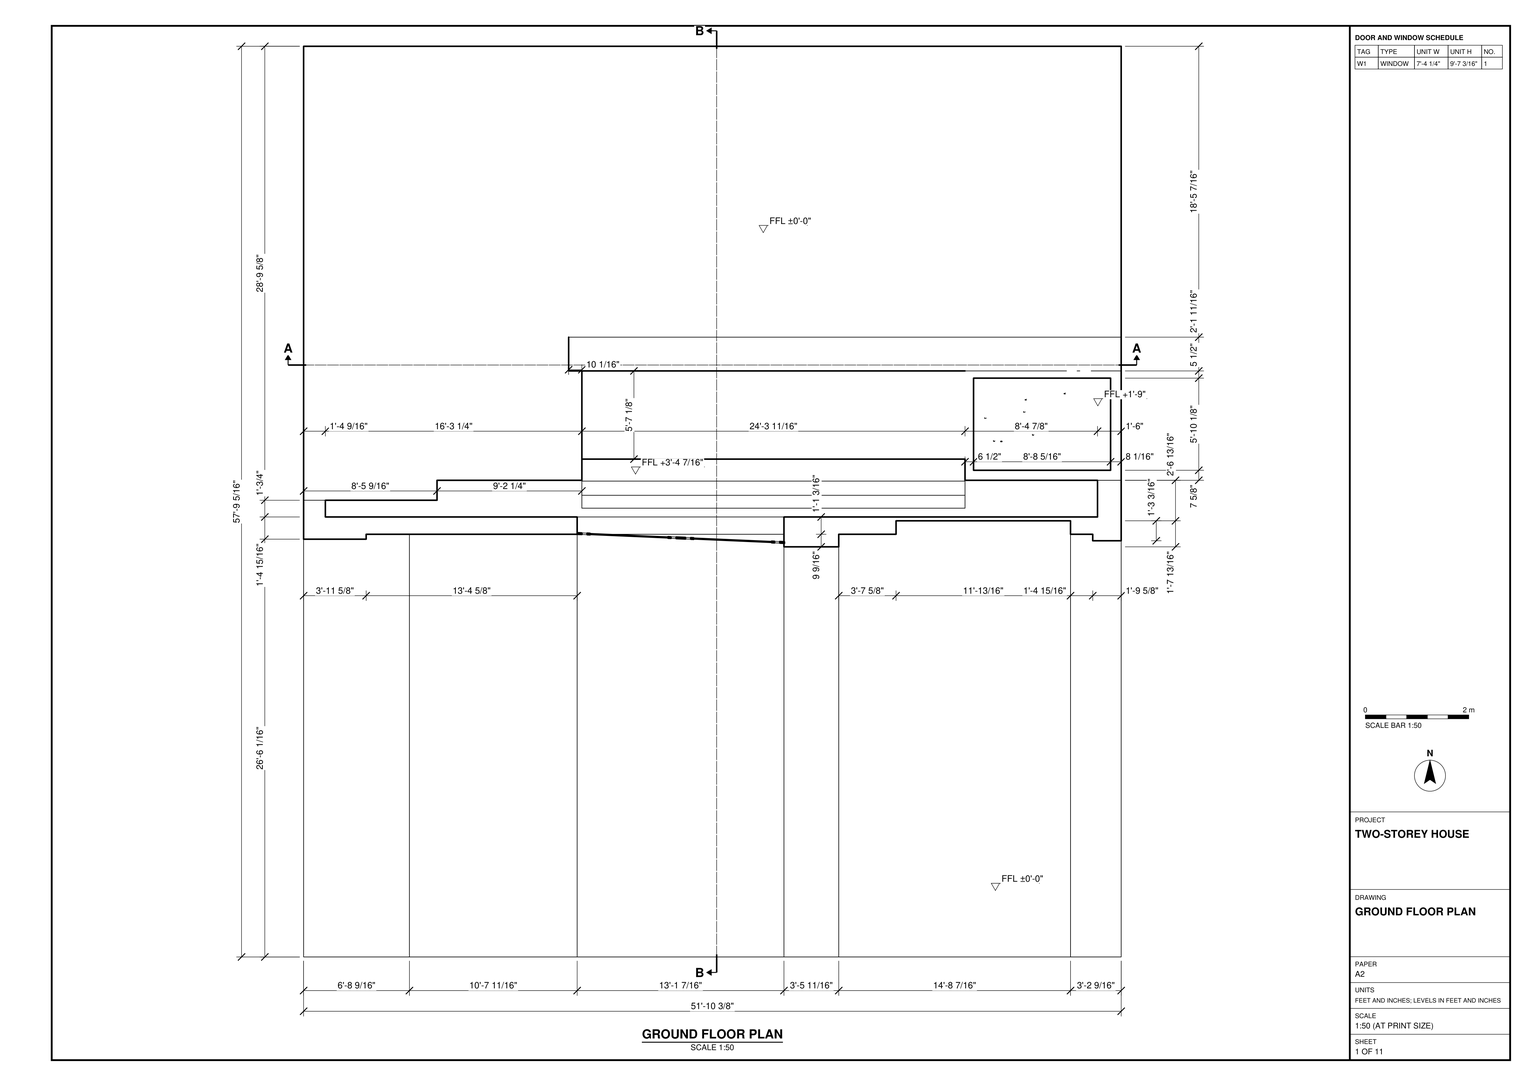
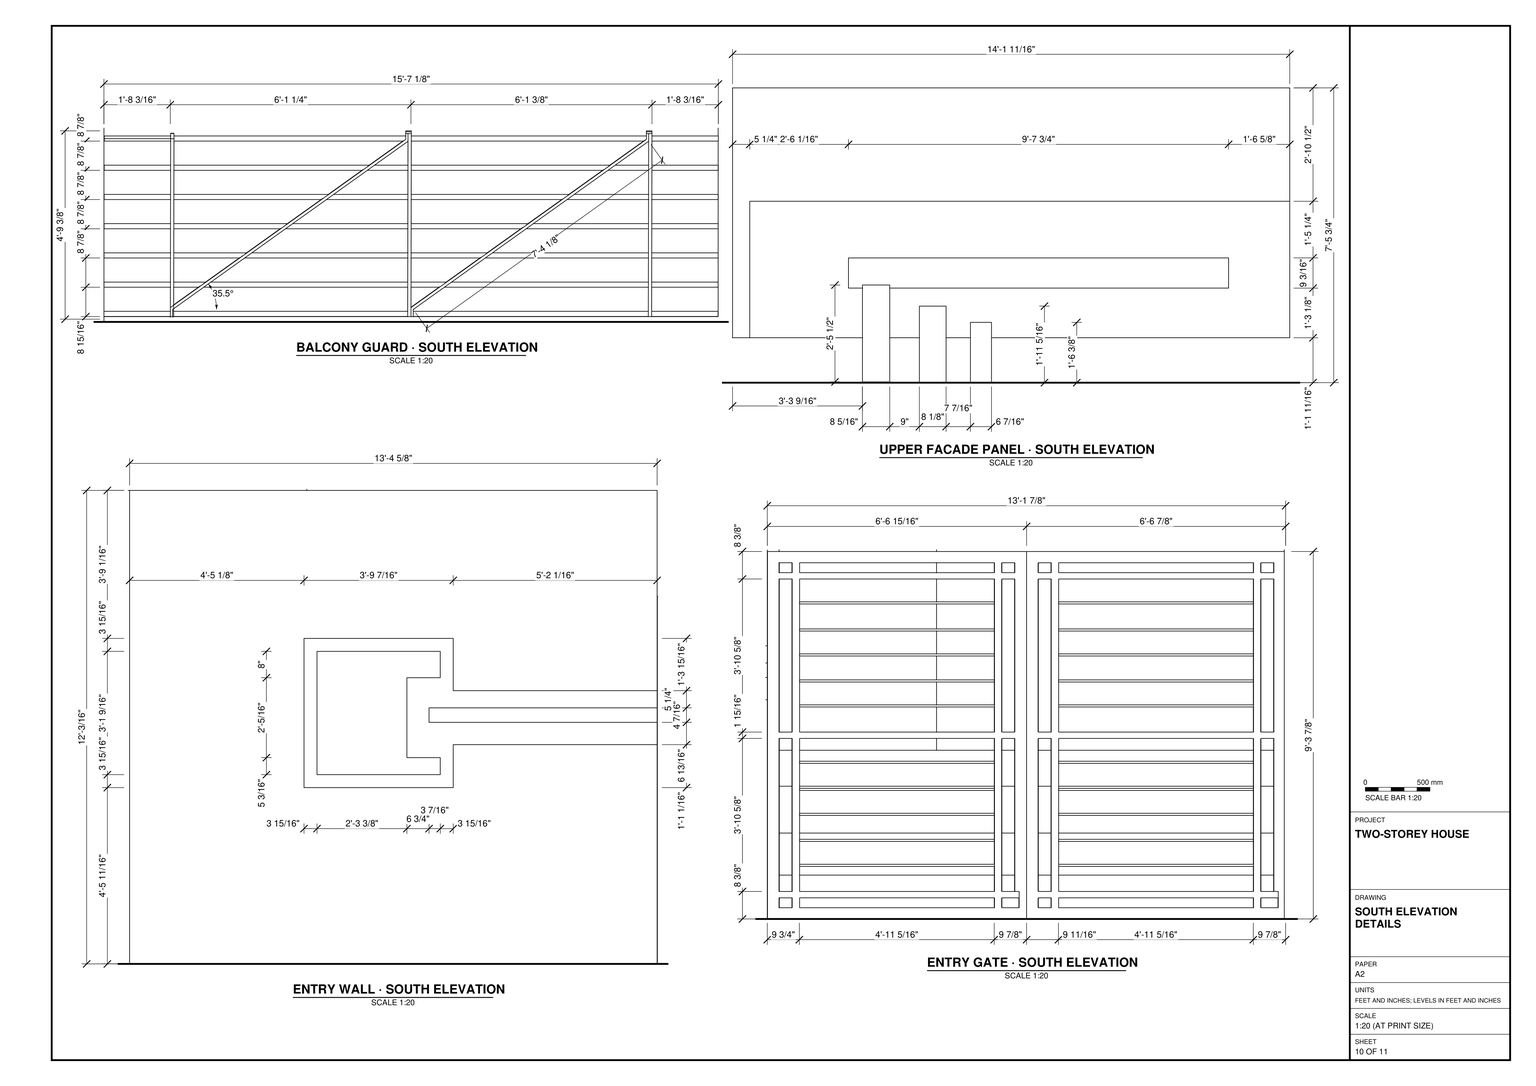
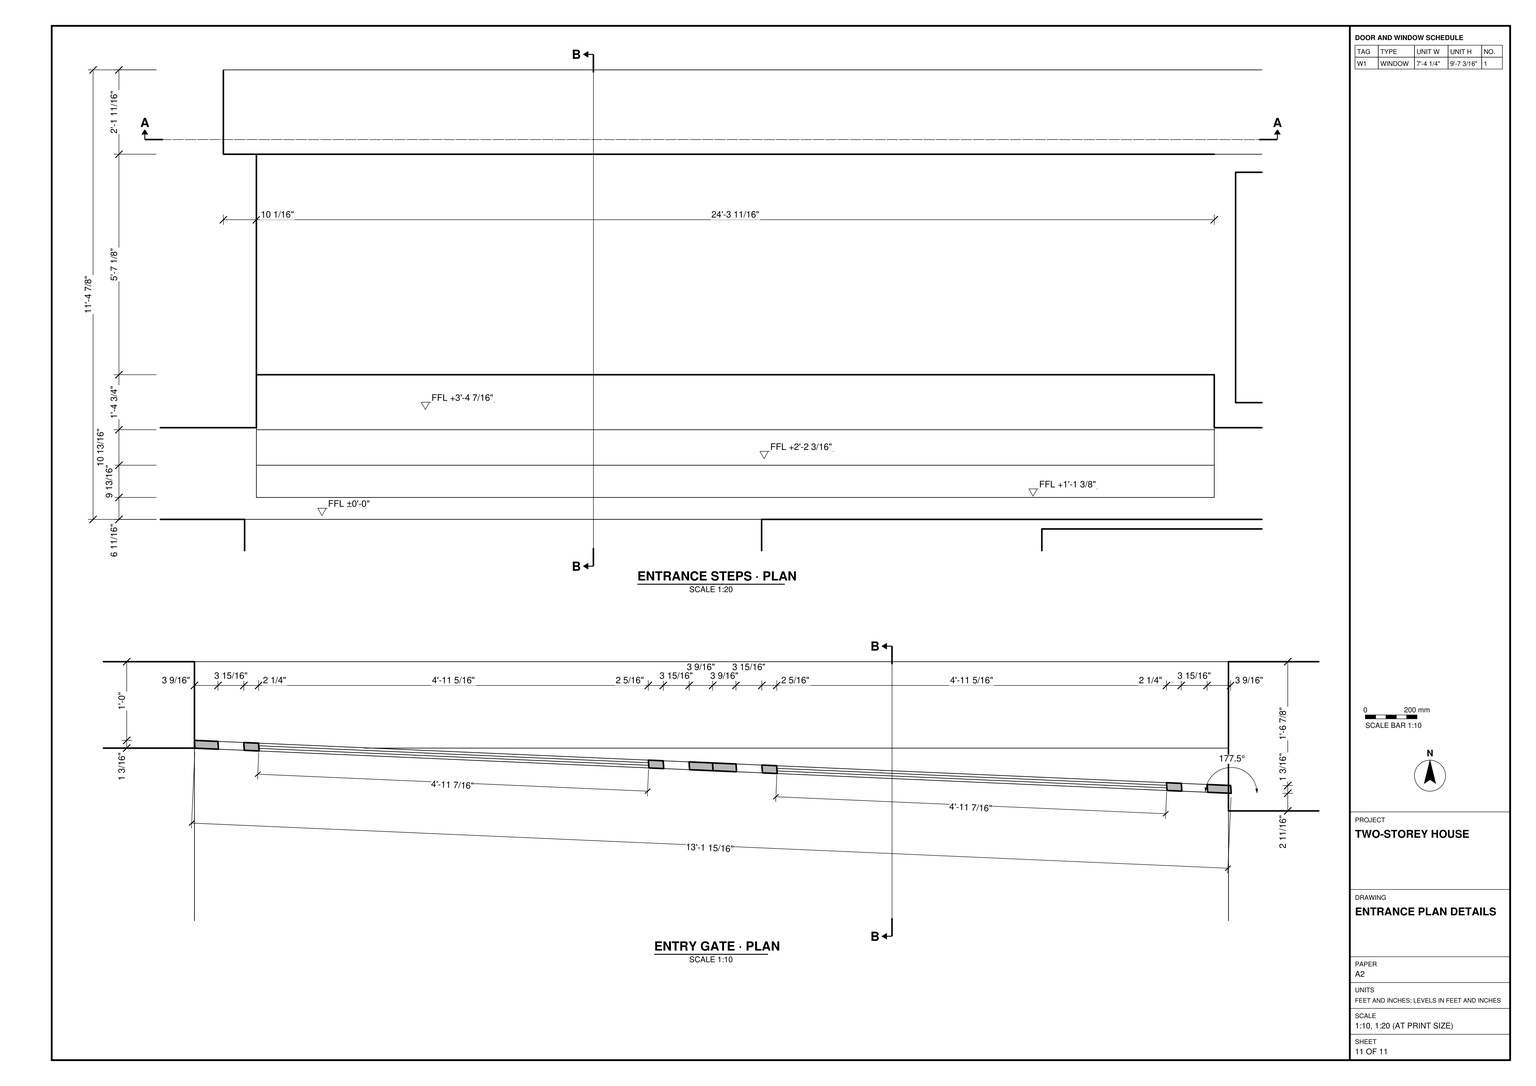
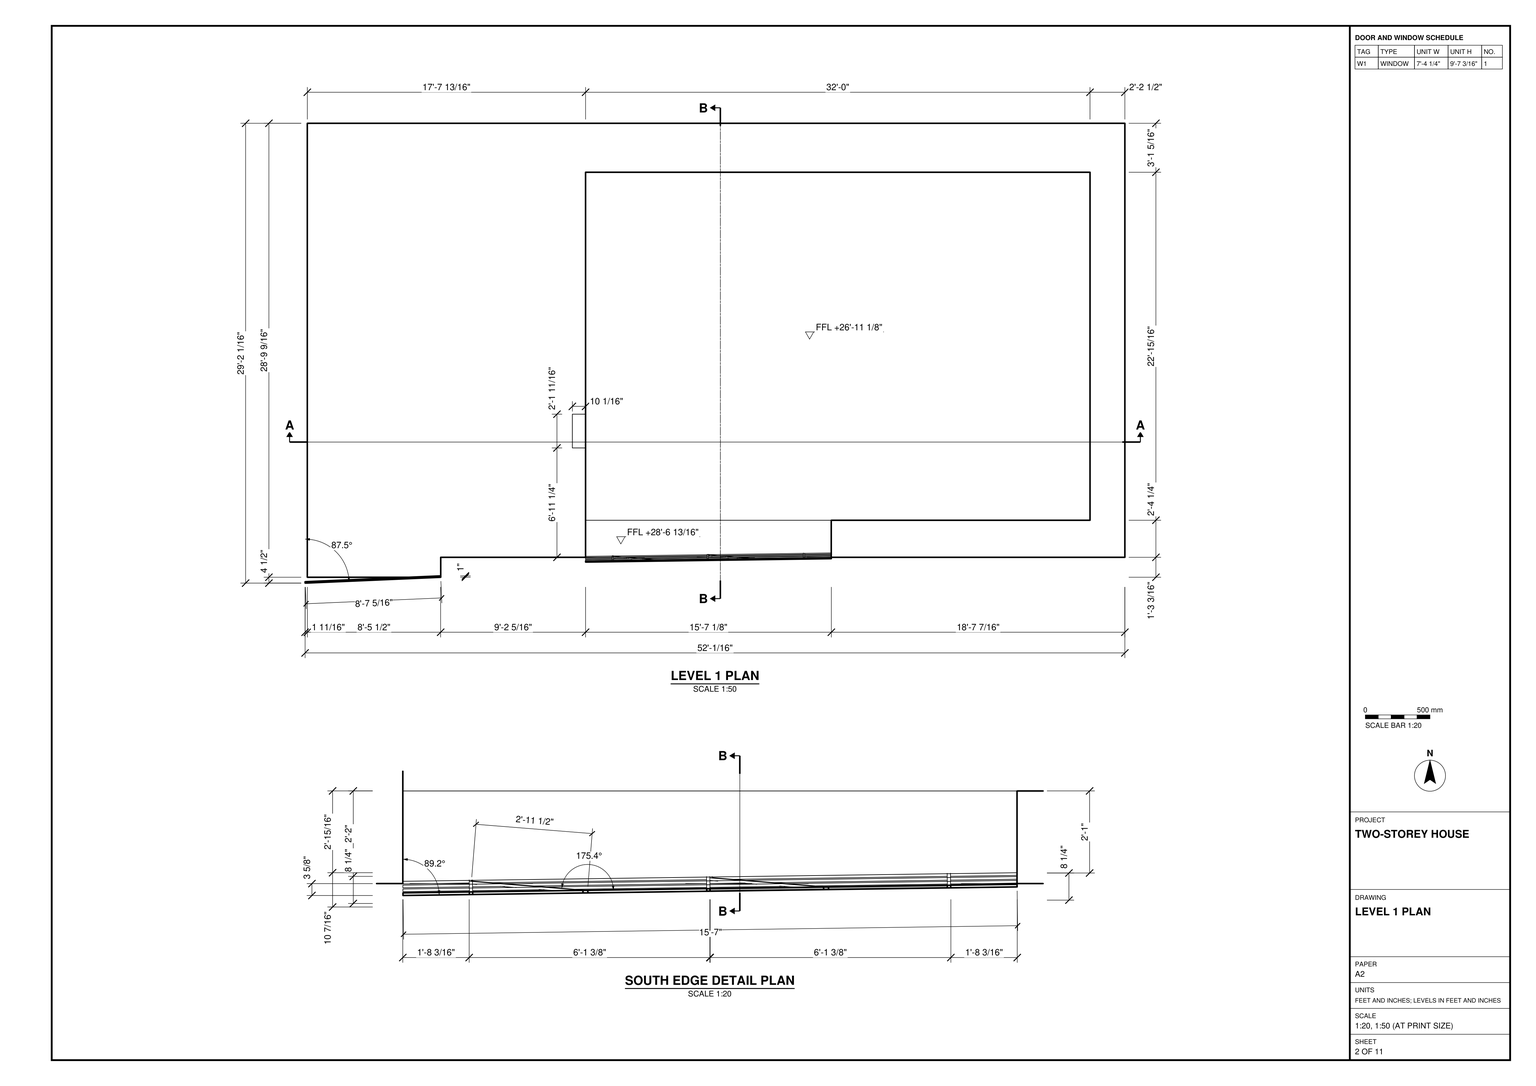
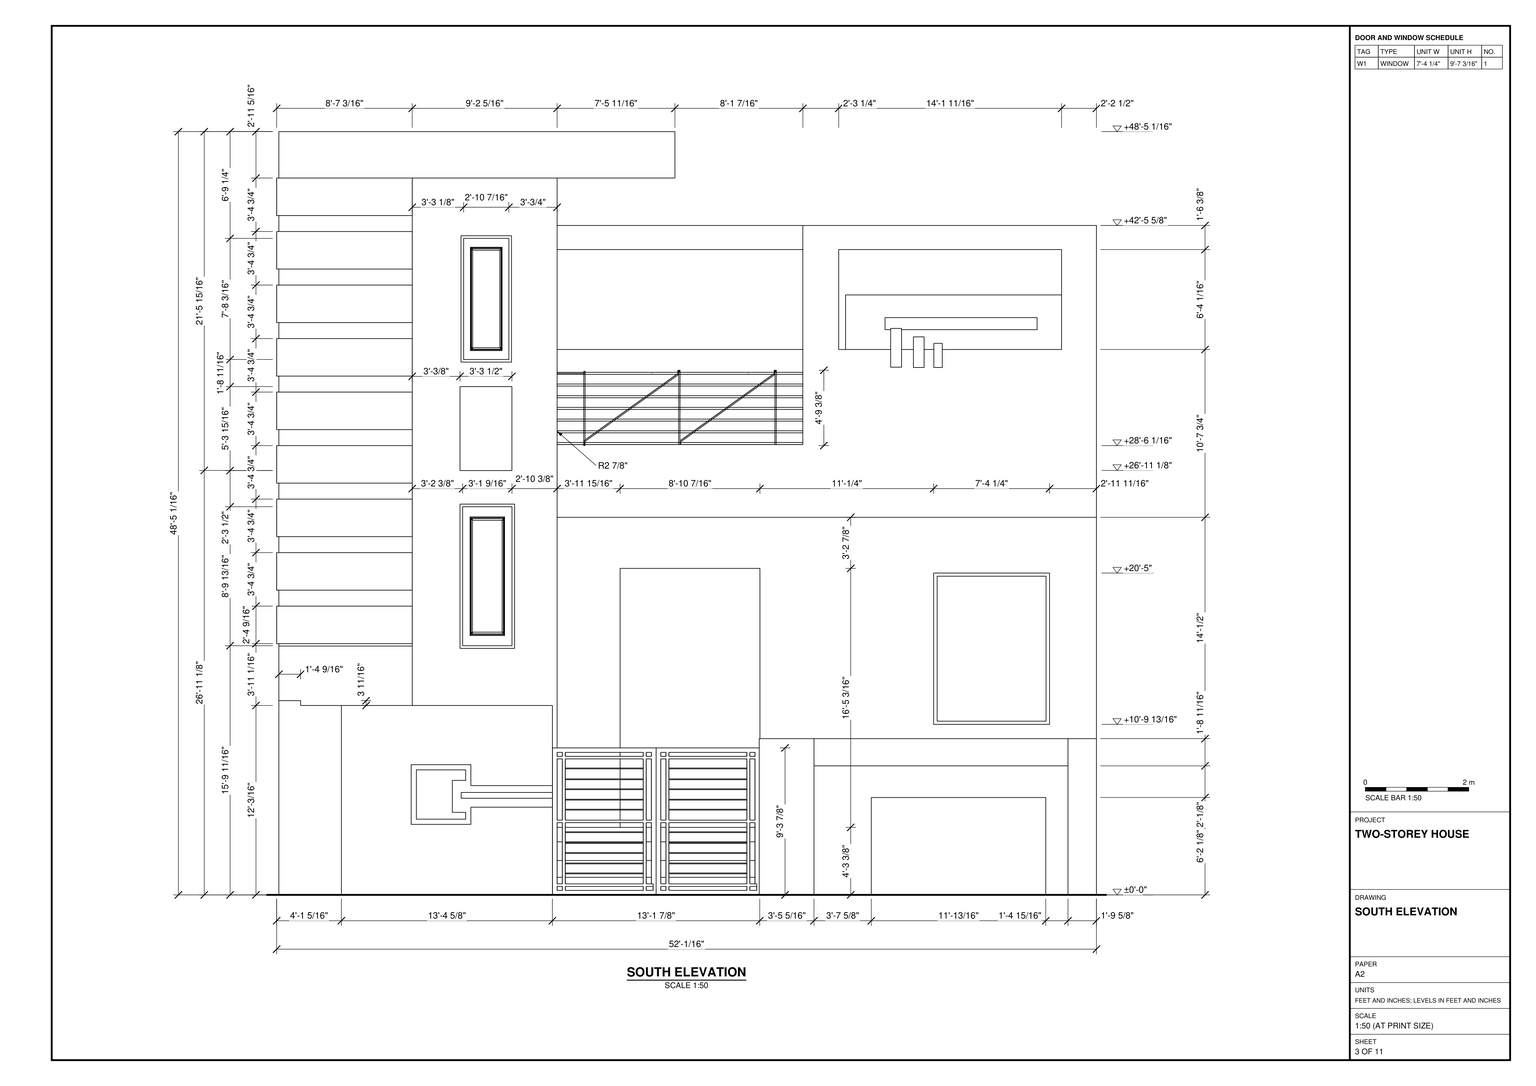
Build the two-storey house and its entrance approach in SketchUp using task_files/diagram_01.pdf. Work in feet and inches. Set out the complete model to an overall width of 52'-8 1/4" along X, a depth of 57'-9 5/16" along Y and a height of 48'-5 1/16" along Z. Use ±0'-0" for the ground floor and +26'-11 1/8" for the upper floor.

Use the plans and sections to place the walls at their drawn thicknesses, fit the openings and window unit, and form the slabs, balcony and roof. At the south entrance, preserve the open approach in front of the gate. Set the gate at the slight angle shown in plan, and model its two framed leaves with horizontal slats. Behind the gate, form the broad run of steps up to the raised landing. Reproduce the outlined rectangular motif and horizontal bands on the entry wall. Use the elevation details to lay out the balcony guard, including its horizontal rails and diagonal braces, and the separate upper facade panel.

Keep shell elements such as walls, slabs and roof, and each furniture or joinery piece shown, in separate groups or components. Use components for repeated parts. Decor and loose items may be represented by any suitable library components. Save one SketchUp model as output_files/two_storey_house_with_its_gated_entrance_and_balcony.skp.

# SketchUp Ruby script. Lengths in inches.
U = 1.inch
M = Sketchup.active_model
def pt(a) = Geom::Point3d.new(a.map { |v| v * U })
def face(e, loops, mat)
  f = e.add_face(loops[0].map { |a| pt(a) })
  loops[1..].each { |l| e.add_face(l.map { |a| pt(a) }).erase! }
  f.material = f.back_material = mat if mat
  f
end
# faces: each face lists its corners as indices into pts; further lists are holes
def faces(e, pts, list, mat = nil) = list.each { |f| face(e, (f[0].is_a?(Array) ? f : [f]).map { |l| l.map { |i| pts[i] } }, mat) }
# xy, xz, yz: faces in a plane at the given z, y or x. An outline is a flat list of corners, or four numbers for a rectangle; further outlines are holes
def ring(l) = l.size == 4 ? [[l[0], l[1]], [l[2], l[1]], [l[2], l[3]], [l[0], l[3]]] : l.each_slice(2).to_a
def flat(e, list, mat, &to3) = list.each { |f| face(e, (f[0].is_a?(Array) ? f : [f]).map { |l| ring(l).map { |u, v| to3.(u, v) } }, mat) }
def xy(e, z, list, mat = nil) = flat(e, list, mat) { |x, y| [x, y, z] }
def xz(e, y, list, mat = nil) = flat(e, list, mat) { |x, z| [x, y, z] }
def yz(e, x, list, mat = nil) = flat(e, list, mat) { |y, z| [x, y, z] }
def lines(e, pts, list) = list.each { |a, b| e.add_line(pt(pts[a]), pt(pts[b])) }
# prism: a flat outline (further loops are holes) pulled along v
def prism(e, loops, v, mat = nil)
  f = face(e, loops, mat); d = Geom::Vector3d.new(v.map { |x| x * U })
  f.pushpull(f.normal.samedirection?(d) ? d.length : -d.length)
end
def box(e, o, s, mat = nil) = prism(e, [[o, [o[0] + s[0], o[1], o[2]], [o[0] + s[0], o[1] + s[1], o[2]], [o[0], o[1] + s[1], o[2]]]], [0, 0, s[2]], mat)
def at(x, y, z, deg = 0) = Geom::Transformation.translation(pt([x, y, z])) * Geom::Transformation.rotation(ORIGIN, Z_AXIS, deg.degrees)
def axes(o, x, y, z) = Geom::Transformation.new([*x, 0, *y, 0, *z, 0, *pt(o).to_a, 1])
def part(name) = M.definitions.add(name)
# library, detail: a bought-in or finely detailed component or shape, given as its bounding box
def library(name, o, s) = part(name).tap { |d| box(d.entities, o, s) }
def detail(e, o, s) = box(e.add_group.entities, o, s)
def put(e, d, t, mat = nil) = e.add_instance(d, t).tap { |i| i.material = mat if mat }
def group(e, t, mat = nil) = e.add_group.tap { |g| g.transformation = t; g.material = mat if mat }.entities
root = M.entities
M.materials.add("Niraj_Shoe_Sole").color = [96, 73, 48]
M.materials.add("Niraj_Shoe_Stitching").color = [181, 137, 92]
M.materials.add("[0038_Orange]").color = [255, 165, 0]
M.materials.add("[0043_SaddleBrown]").color = [139, 69, 19]
M.materials.add("[0136_Charcoal]").color = [35, 35, 35]
M.materials.add("[Asphalt New]").color = [67, 60, 62]
M.materials.add("[Color B07]").color = [153, 38, 0]
M.materials.add("[Color C08]").color = [58, 29, 0]
M.materials.add("[Concrete Block Layers]").color = [147, 139, 140]
M.materials.add("[Rough Square Concrete Block]").color = [123, 120, 113]
M.materials.add("[Translucent Glass Gray]").color = [128, 128, 128]
M.materials["[Translucent Glass Gray]"].alpha = 0.5
M.materials.add("[Translucent_Glass_Blue]").color = [68, 104, 165]
M.materials["[Translucent_Glass_Blue]"].alpha = 0.07
M.materials.add("[Translucent_Glass_Green_Dark]").color = [33, 68, 103]
M.materials["[Translucent_Glass_Green_Dark]"].alpha = 0.08
M.materials.add("hymenocallis littoralis").color = [156, 172, 146]
c1 = library("grille P1",[0,0,0],[0.79,28.9,72.83])
c2 = part("Framed panel")
xy(c2.entities,0,[[0,0,20,1.125]],"[Color C08]")
xy(c2.entities,3,[[3,0,17,0.5625],[3,0.5625,17,1.125]])
xy(c2.entities,38,[[3,0,17,0.5625],[3,0.5625,17,1.125]])
xy(c2.entities,41,[[0,0,20,1.125]],"[Color C08]")
xz(c2.entities,0,[[[0,0,20,41],[3,3,17,38]]],"[Color C08]")
xz(c2.entities,0.5625,[[3,3,4,4],[4,3,17,4],[3,4,4,38],[16,4,17,37],[4,37,17,38]])
xz(c2.entities,0.5625,[[4,4,16,37]],"[Translucent Glass Gray]")
xz(c2.entities,1.125,[[[0,0,20,41],[3,3,17,38]]])
yz(c2.entities,0,[[0,0,1.125,41]],"[Color C08]")
yz(c2.entities,3,[[0,3,0.5625,38],[0.5625,3,1.125,38]])
yz(c2.entities,17,[[0,3,0.5625,38],[0.5625,3,1.125,38]])
yz(c2.entities,20,[[0,0,1.125,41]],"[Color C08]")
p = [[3,0,3],[3.25,0.14,3.25],[16.75,0.14,3.25],[17,0,3],[3,0,38],[3.25,0.14,37.75],
  [16.75,0.14,37.75],[17,0,38],[3.5,0.28,3.5],[3.5,0.28,37.5],[16.5,0.28,3.5],[16.5,0.28,37.5],
  [16,0.5625,4],[4,0.5625,4],[4,0.5625,37],[4,0.5625,5],[16,0.5625,37]]
faces(c2.entities,p,[[0,1,2,3],[4,5,1,0],[3,2,6,7],[8,1,5,9],[10,2,1,8],[11,6,2,10],[12,10,8,13],[13,8,9,14,15],
  [16,11,10,12],[14,9,11,16],[9,5,6,11],[7,6,5,4]],"[Color C08]")
c3 = library("Double entrance gate",[0,0,0],[87.31,5.6,111.9])
c4 = part("DOOR12")
g1 = group(c4.entities,at(114.73,28.14,-0.51))
g2 = group(g1,at(0,0,0))
box(g2,[0,0,0],[36,0.5,77.7])
c5 = part("Two-panel window \#1")
xy(c5.entities,-18,[[0,-31,2,35]],"[0136_Charcoal]")
xy(c5.entities,-16,[[0,-29,0.9375,33],[0.9375,-29,1.125,33],[1.125,-29,2,1],[1.125,3,2,33]],"[0136_Charcoal]")
xy(c5.entities,76,[[0,-29,0.9375,33],[0.9375,-29,1.125,33],[1.125,-29,2,1],[1.125,3,2,33]],"[0136_Charcoal]")
xy(c5.entities,78,[[0,-31,2,35]],"[0136_Charcoal]")
xz(c5.entities,-31,[[0,-18,2,78]],"[0136_Charcoal]")
xz(c5.entities,-29,[[0,-16,0.9375,76],[0.9375,-16,1.125,76],[1.125,-16,2,76]],"[0136_Charcoal]")
xz(c5.entities,1,[[1.125,-16,2,76]],"[0136_Charcoal]")
xz(c5.entities,3,[[1.125,-16,2,76]],"[0136_Charcoal]")
xz(c5.entities,33,[[0,-16,0.9375,76],[0.9375,-16,1.125,76],[1.125,-16,2,76]],"[0136_Charcoal]")
xz(c5.entities,35,[[0,-18,2,78]],"[0136_Charcoal]")
yz(c5.entities,0,[[[-31,-18,35,78],[-29,-16,33,76]]],"[0136_Charcoal]")
yz(c5.entities,0.9375,[[-29,-16,33,76]],"[Translucent_Glass_Blue]")
yz(c5.entities,1.125,[[1,-16,3,76]],"[0136_Charcoal]")
yz(c5.entities,1.125,[[-29,-16,1,76],[3,-16,33,76]],"[Translucent_Glass_Green_Dark]")
yz(c5.entities,2,[[[-31,-18,35,78],[-29,-16,1,76],[3,-16,33,76]]],"[0136_Charcoal]")
c6 = part("Two-panel window")
put(c6.entities,c5,axes([-31.84,50.72,0],[1,0,0],[0,1.1,0],[0,0,1]))
c7 = part("normal+window")
put(c7.entities,c6,axes([114.26,44.3125,18],[0,1,0],[-0.90909,0,0],[0,0,1]))
c8 = part("Group\#856")
xy(c8.entities,7.38,[[0,0,5.5,15.91]],"hymenocallis littoralis")
p = [[5.5,28.78,0],[5.5,26.79,3.44],[0,26.79,3.44],[0,28.78,0],[0,23.75,6],[5.5,23.75,6],
  [0,15.91,7.38],[5.5,15.91,7.38]]
faces(c8.entities,p,[[0,1,2,3],[4,2,1,5],[6,4,5,7]],"hymenocallis littoralis")
c9 = part("Group\#854")
xy(c9.entities,7.38,[[0,0,5.5,15.91],[0,15.91,5.5,23.87]],"hymenocallis littoralis")
p = [[5.5,31.07,4.3],[5.5,27.74,6.47],[0,27.74,6.47],[0,31.07,4.3],[0,23.87,7.38],[5.5,23.87,7.38]]
faces(c9.entities,p,[[0,1,2,3],[4,2,1,5]],"hymenocallis littoralis")
c10 = part("Group\#857")
xy(c10.entities,7.38,[[0,0,5.6,15.91]],"hymenocallis littoralis")
p = [[5.6,28.78,0],[5.6,26.79,3.44],[0,26.79,3.44],[0,28.78,0],[0,23.75,6],[5.6,23.75,6],
  [0,15.91,7.38],[5.6,15.91,7.38]]
faces(c10.entities,p,[[0,1,2,3],[4,2,1,5],[6,4,5,7]],"hymenocallis littoralis")
c11 = part("Group\#855")
put(c11.entities,c9,axes([6.09,8.57,-0.52],[0.446,0.85617,0.26089],[-0.18444,-0.19731,0.96283],[0.87582,-0.47754,0.0699]))
put(c11.entities,c9,axes([6.29,7.28,-1.71],[0.37058,0.92707,-0.05667],[-0.32382,0.19004,0.99128],[0.87712,-0.32925,0.34964]))
put(c11.entities,c9,axes([11.04,16.14,-0.7],[1,0,0],[0,0.16628,1.02662],[0,-1.18456,0.19186]))
c12 = part("Group\#860")
put(c12.entities,c8,axes([24.57,32.05,-1.76],[0.9552,-0.22102,-0.19681],[0.4036,0.95545,0.88585],[-0.00568,-0.67859,0.7345]))
put(c12.entities,c8,axes([23.95,29.24,-2.4],[0,1,0],[-0.76041,0,0.64945],[0.64945,0,0.76041]))
put(c12.entities,c8,axes([24.22,24.72,-0.48],[-0.70711,0.70711,0],[-0.32757,-0.32757,0.80237],[0.61237,0.61237,0.5]))
put(c12.entities,c9,axes([20.66,37.22,-0.63],[1.12361,0.03262,0.39091],[-0.43499,0.29739,0.78777],[0.09852,-1.27434,0.37535]))
put(c12.entities,c8,axes([28.75,24.45,-2.4],[-1,0,0],[0,-0.76041,0.64945],[0,0.64945,0.76041]))
put(c12.entities,c10,axes([30.4,30.98,-3.7],[0.65676,-0.72002,0.22414],[0.55667,0.66341,0.5],[-0.50871,-0.20361,0.83652]))
put(c12.entities,c10,axes([32.41,29.61,-3.7],[0.04029,-0.97372,0.22414],[0.85287,0.15038,0.5],[-0.52057,0.17102,0.83652]))
put(c12.entities,c8,axes([31.89,25.85,-1.76],[-0.92056,0.33739,-0.19681],[-0.5186,-0.89824,0.88585],[0.08952,0.67268,0.7345]))
put(c12.entities,c8,axes([25.55,34.78,-0.48],[0.86603,0.5,0],[-0.25,0.43301,0.86603],[0.43301,-0.75,0.5]))
put(c12.entities,c10,axes([20.4,16.9375,-8.07],[-0.70711,0.70711,0],[-0.35754,-0.35754,0.65422],[1.3987,1.3987,1.52882]))
put(c12.entities,c8,axes([32.86,34.14,-0.48],[0.76604,-0.64279,0],[0.32139,0.38302,0.86603],[-0.55667,-0.66341,0.5]))
put(c12.entities,c8,axes([27.15,34.7,-0.1],[0.82472,-0.17528,-0.53769],[0.53769,0.53769,0.64945],[0.17528,-0.82472,0.53769]))
put(c12.entities,c8,axes([33.58,28.77,-2.4],[0,-1,0],[0.76041,0,0.64945],[-0.64945,0,0.76041]))
put(c12.entities,c8,axes([26.43,23.87,-2.81],[-0.75126,0.04415,0.65853],[0.53769,-0.53769,0.64945],[0.38276,0.84199,0.3802]))
put(c12.entities,c8,axes([28.78,23.98,-2.4],[-1,0,0],[0,-0.76041,0.64945],[0,0.64945,0.76041]))
put(c12.entities,c8,axes([25.39,25.38,-2.4],[-0.70711,0.70711,0],[-0.53769,-0.53769,0.64945],[0.45923,0.45923,0.76041]))
put(c12.entities,c8,axes([27.32,21.63,-0.1],[-0.45923,0.70711,-0.53769],[-0.76041,0,0.64945],[0.45923,0.70711,0.53769]))
put(c12.entities,c8,axes([25.17,27.625,-1.76],[0.56416,0.80187,-0.19681],[-0.66673,0.66673,0.80532],[0.62659,-0.26057,0.7345]))
put(c12.entities,c10,axes([27.59,27.04,-3.96],[-0.8993,-0.06127,0.43301],[0.2962,-0.8138,0.5],[0.32175,0.57791,0.75]))
put(c12.entities,c10,axes([26.98,24.5,-3.18],[-0.5,0.86603,0],[-0.75,-0.43301,0.5],[0.43301,0.25,0.86603]))
put(c12.entities,c10,axes([24.55,27.74,-3.7],[0.29517,0.92878,0.22414],[-0.85287,0.15038,0.5],[0.43068,-0.33875,0.83652]))
put(c12.entities,c10,axes([24.26,29.8,-3.18],[0.76604,0.64279,0],[-0.47317,0.5639,0.425],[0.32139,-0.38302,0.86603]))
put(c12.entities,c10,axes([25.98,32.46,-3.18],[1,0,0],[0,0.86603,0.5],[0,-0.5,0.86603]))
put(c12.entities,c8,axes([28.78,33.57,-2.4],[1,0,0],[0,0.76041,0.64945],[0,-0.64945,0.76041]))
put(c12.entities,c11,at(14.99,21.38,2.5))
put(c12.entities,c9,axes([34.63,26.34,-1.46],[-0.70089,-0.70877,0.07994],[0.4756,-0.38088,0.79293],[-0.53156,0.59378,0.60405]))
put(c12.entities,c9,axes([28.14,16.92,1.8125],[-1.19719,0.6912,0],[-0.09607,-0.16641,0.94244],[0.68444,1.18549,0.17613]))
put(c12.entities,c9,axes([31.5625,35.84,0.97],[0.66765,-1.1564,0.35779],[0.04445,0.30732,0.91033],[-1.20828,-0.64496,0.17012]))
put(c12.entities,c9,axes([38.94,22.51,0.89],[-0.97932,-0.67164,-0.05202],[0.27787,-0.41401,0.90999],[-0.85985,0.93577,0.32097]))
put(c12.entities,c9,axes([38.44,21.09,1.98],[-1.02864,-0.54856,0.2395],[0.33481,0.06999,0.88388],[-0.77261,1.08328,0.06417]))
put(c12.entities,c10,axes([35.02,30.51,-1.3],[-0.17365,-0.98481,0],[0.60224,-0.10619,0.79122],[-0.7792,0.13739,0.61153]))
put(c12.entities,c10,axes([29.41,22.33,-1.3],[-0.93969,0.34202,0],[-0.20915,-0.57465,0.79122],[0.27061,0.74351,0.61153]))
put(c12.entities,c9,axes([19.64,36,-1.62],[1.18194,0.09546,0.08234],[-0.14377,0.68823,0.76313],[0.21457,-1.1326,0.62386]))
put(c12.entities,c10,axes([24.25,24.14,-1.3],[-0.34202,0.93969,0],[-0.57465,-0.20915,0.79122],[0.74351,0.27061,0.61153]))
put(c12.entities,c10,axes([25.98,34.61,-1.3],[1,0,0],[0,0.61153,0.79122],[0,-0.79122,0.61153]))
put(c12.entities,c10,axes([31.16,34.41,-1.64],[0.56518,-0.80224,-0.19234],[0.73413,0.34233,0.72935],[-0.47639,-0.50772,0.71782]))
put(c12.entities,c10,axes([40.52,26.84,-5.82],[-0.42262,-0.90631,0],[0.48019,-0.22391,0.68552],[-1.43418,0.66877,1.22305]))
put(c12.entities,c8,axes([29.86,38.42,-1.01],[0.89064,-0.37013,0.26413],[-0.03924,0.63286,1.01918],[-0.45353,-0.76487,0.45748]))
put(c12.entities,c8,axes([29.34,22.4,-0.48],[-0.99619,-0.08716,0],[0.04358,-0.4981,0.86603],[-0.07548,0.86273,0.5]))
c13 = part("Group\#858")
xz(c13.entities,10.07,[[9.07,0,10.07,31.01],[0,31.01,0,45.12,20.13,45.12,20.13,31.01,10.07,31.01,10.07,32.58,9.07,32.58,9.07,31.01]],"hymenocallis littoralis")
yz(c13.entities,10.07,[[0,31.01,20.13,45.12]],"hymenocallis littoralis")
p = [[9.57,9.2,0],[10.07,10.07,0],[10.07,10.07,31.01],[10.07,10.07,32.58],[9.57,9.2,32.58]]
faces(c13.entities,p,[[0,1,2,3,4]],"hymenocallis littoralis")
c14 = part("cây lá nắng")
put(c14.entities,c12,axes([49.26,-2.75,0],[0.63109,0.63109,0],[-0.63109,0.63109,0],[0,0,0.935]))
g3 = group(c14.entities,at(26.6,-8.68,0))
put(g3,c8,axes([-4.72,35.73,-1.65],[0.74231,0.46334,-0.18402],[-0.34827,0.85768,0.82827],[0.42467,-0.43184,0.68675]))
put(g3,c8,axes([-3.34,33.57,-2.24],[-0.63109,0.63109,0],[-0.47989,-0.47989,0.60723],[0.40986,0.40986,0.71098]))
put(g3,c8,axes([-0.3125,30.89,-0.45],[-0.8925,0,0],[0,-0.41345,0.75022],[0,0.77293,0.4675]))
put(g3,c9,axes([-10.79,39.66,-0.59],[0.68852,0.72969,0.3655],[-0.4622,-0.08684,0.73657],[0.86641,-0.74205,0.35095]))
put(g3,c8,axes([2.71,33.57,-2.24],[-0.63109,-0.63109,0],[0.47989,-0.47989,0.60723],[-0.40986,0.40986,0.71098]))
put(g3,c10,axes([-0.37,38.74,-3.46],[0.86887,-0.03992,0.20957],[-0.06737,0.76999,0.4675],[-0.19255,-0.44954,0.78214]))
put(g3,c10,axes([1.76,39.14,-3.46],[0.63993,-0.58908,0.20957],[0.44333,0.63315,0.4675],[-0.43646,-0.2206,0.78214]))
put(g3,c8,axes([3.81,36.4375,-1.65],[-0.79389,-0.36803,-0.18402],[0.23959,-0.89415,0.82827],[-0.36803,0.48102,0.68675]))
put(g3,c8,axes([-5.83,38.07,-0.45],[0.231,0.86209,0],[-0.43104,0.1155,0.80973],[0.74659,-0.20005,0.4675]))
put(g3,c10,axes([2.18,23.5625,-7.55],[-0.8925,0,0],[0,-0.45128,0.6117],[0,1.76542,1.42944]))
put(g3,c8,axes([-0.8125,42.28,-0.45],[0.8891,0.07779,0],[-0.03889,0.44455,0.80973],[0.06737,-0.76999,0.4675]))
put(g3,c8,axes([-4.76,39.03,-0.09],[0.63109,0.40986,-0.50274],[0,0.67866,0.60723],[0.63109,-0.40986,0.50274]))
put(g3,c8,axes([3.03,39.35,-2.24],[0.63109,-0.63109,0],[0.47989,0.47989,0.60723],[-0.40986,-0.40986,0.71098]))
put(g3,c8,axes([1.61,31.74,-2.625],[-0.50198,-0.44625,0.61573],[0.67866,0,0.60723],[-0.28982,0.77293,0.35549]))
put(g3,c8,axes([3.03,33.3,-2.24],[-0.63109,-0.63109,0],[0.47989,-0.47989,0.60723],[-0.40986,0.40986,0.71098]))
put(g3,c8,axes([0.01,32.04,-2.24],[-0.8925,0,0],[0,-0.67866,0.60723],[0,0.57963,0.71098]))
put(g3,c8,axes([3.59,30.89,-0.09],[-0.73607,0.15643,-0.50274],[-0.47989,-0.47989,0.60723],[-0.15643,0.73607,0.50274]))
put(g3,c8,axes([-1.55,33.32,-1.65],[-0.15002,0.86209,-0.18402],[-0.84154,0,0.75297],[0.55988,0.231,0.68675]))
put(g3,c10,axes([0.35,34.48,-3.71],[-0.52887,-0.60621,0.40487],[0.70051,-0.32665,0.4675],[-0.16166,0.56777,0.70125]))
put(g3,c10,axes([2.61,39.13,-1.74],[-0.86209,0.231,0],[-0.23031,-0.85954,0.15531],[0.03162,0.11799,0.91645]))
put(g3,c10,axes([-2.02,33,-3.46],[-0.39986,0.77243,0.20957],[-0.63315,-0.44333,0.4675],[0.48558,0.05802,0.78214]))
put(g3,c10,axes([-3.49,34.12,-2.97],[0.07779,0.8891,0],[-0.65449,0.05726,0.39737],[0.44455,-0.03889,0.80973]))
put(g3,c10,axes([-4.09,36.88,-2.97],[0.63109,0.63109,0],[-0.54654,0.54654,0.4675],[0.31555,-0.31555,0.80973]))
put(g3,c8,axes([-3.02,39.35,-2.24],[0.63109,0.63109,0],[-0.47989,0.47989,0.60723],[0.40986,-0.40986,0.71098]))
put(g3,c11,axes([-4.03,22.95,2.33],[0.63109,0.63109,0],[-0.63109,0.63109,0],[0,0,0.935]))
put(g3,c9,axes([5.24,38.48,-1.37],[0.00497,-0.88963,0.07474],[0.54052,0.05978,0.74139],[-0.71019,0.03927,0.56479]))
put(g3,c9,axes([7.08,28.4375,1.7],[-1.19175,-0.31933,0],[0.04439,-0.16565,0.88118],[-0.31621,1.1801,0.16468]))
put(g3,c9,axes([-2.7,42.54,0.91],[1.15114,-0.30845,0.33454],[-0.1659,0.22199,0.85115],[-0.3555,-1.16957,0.15907]))
put(g3,c9,axes([10.37,38.78,0.83],[-0.19417,-1.04191,-0.04864],[0.43664,-0.08592,0.85084],[-1.1332,0.04791,0.30011]))
put(g3,c9,axes([10.95,37.5625,1.85],[-0.30298,-0.99536,0.22393],[0.16713,0.25547,0.82643],[-1.17124,0.19607,0.06]))
put(g3,c10,axes([2.84,41.36,-1.22],[0.51192,-0.73109,0],[0.44708,0.31305,0.73979],[-0.57846,-0.40504,0.57178]))
put(g3,c10,axes([4.47,32.65,-1.22],[-0.80888,-0.37719,0],[0.23066,-0.49465,0.73979],[-0.29844,0.64,0.57178]))
put(g3,c9,axes([-10.32,35.12,-1.51],[0.68567,0.80616,0.07699],[-0.52507,0.3436,0.71352],[0.85019,-0.57936,0.58331]))
put(g3,c10,axes([0.07,30.54,-1.22],[-0.80888,0.37719,0],[-0.23066,-0.49465,0.73979],[0.29844,0.64,0.57178]))
put(g3,c10,axes([-5.45,38.24,-1.22],[0.63109,0.63109,0],[-0.38593,0.38593,0.73979],[0.49934,-0.49934,0.57178]))
put(g3,c10,axes([-2.05,41.38,-1.53],[0.86296,-0.14961,-0.17984],[0.24726,0.67935,0.68194],[0.01977,-0.62107,0.67116]))
put(g3,c10,axes([8.63,42.51,-5.4375],[0.30525,-0.83868,0],[0.44435,0.16173,0.64096],[-1.32716,-0.48305,1.14356]))
put(g3,c8,axes([-5.4,43.09,-0.94],[0.79566,0.32849,0.24696],[-0.42416,0.37462,0.95293],[0.19648,-0.76892,0.42774]))
put(g3,c8,axes([4.38,32.65,-0.45],[-0.57369,-0.68369,0],[0.34185,-0.28684,0.80973],[-0.5921,0.49683,0.4675]))
put(g3,c10,axes([-2,33.84,-0.15],[-0.24601,0.85793,0],[-0.85539,-0.24528,0.15531],[0.11742,0.03367,0.91645]))
put(g3,c10,axes([0.17,30.83,-4.47],[-0.24601,0.85793,0],[-0.85539,-0.24528,0.15531],[0.11742,0.03367,0.91645]))
put(g3,c10,axes([-1.97,32.18,-4.47],[0.58524,0.67383,0],[-0.67184,0.58351,0.15531],[0.09222,-0.0801,0.91645]))
put(g3,c10,axes([-2,34.71,-4.47],[0.88392,-0.12346,0],[0.12309,0.88131,0.15531],[-0.0169,-0.12098,0.91645]))
put(g3,c10,axes([0.11,36.12,-4.47],[0.37822,-0.8084,0],[0.80601,0.37711,0.15531],[-0.11064,-0.05177,0.91645]))
put(c14.entities,c13,axes([29.71,14.29,6.94],[0.425,0.73612,0],[-0.6771,0.39092,-0.33349],[-0.26859,0.15507,0.72712]))
put(c14.entities,c13,axes([42.0625,26.12,6.94],[0.85,0,0],[0,0.78185,-0.33349],[0,0.33349,0.78185]))
put(c14.entities,c12,axes([7.3125,23.0625,0],[0.8925,0,0],[0,0.8925,0],[0,0,0.935]))
put(c14.entities,c13,axes([24.4375,40.23,2.05],[0.85,0,0],[0,0.85,0],[0,0,0.85]))
c15 = part("Planting+101")
put(c15.entities,c14,axes([21.34,32.96,-4.59],[0,-0.71,0],[-0.71,0,0],[0,0,0.71]))
xy(root,115.49,[[367.36,312.23,409.06,312.23,409.06,321.79,452.6875,321.79,452.6875,332.04,585.5,332.04,585.5,321.79,602.41,321.79,602.41,316.85,624.0625,316.85,624.0625,362.88,606.05,362.88,606.05,334.95,367.36,334.95],[1.6875,318.04,49.3,318.04,49.3,321.79,209.92,321.79,209.92,334.95,18.24,334.95,18.24,347.69,1.6875,347.69],[209.92,321.79,367.36,334.95],[18.24,334.95,606.05,334.95,606.05,362.88,505.1875,362.88,505.1875,341.63,213.51,341.63,213.51,362.88,103.25,362.88,103.25,347.69,18.24,347.69],[1.6875,347.69,103.25,347.69,103.25,362.88,213.51,362.88,213.51,446.15,203.45,446.15,203.45,471.83,624.0625,471.83,624.0625,693.29,1.6875,693.29],
  [203.45,446.15,624.0625,471.83]])
xy(root,115.49,[[585.5,0,624.0625,0,624.0625,316.85,602.41,316.85,602.41,321.79,585.5,321.79]],"[Asphalt New]")
xy(root,115.49,[[82.24,0,209.92,321.79],[367.36,0,409.06,312.23]],"[Concrete Block Layers]")
xy(root,115.49,[[1.6875,0,82.24,0,82.24,321.79,49.3,321.79,49.3,318.04,1.6875,318.04],[209.92,0,367.36,321.79],[409.06,0,585.5,0,585.5,332.04,452.6875,332.04,452.6875,321.79,409.06,321.79]],"[Rough Square Concrete Block]")
xy(root,128.86,[[213.51,341.63,505.1875,351.44]])
xy(root,136.49,[[511.6875,370.5,616,440.65]])
xy(root,141.65,[[213.51,351.44,505.1875,362.25]])
xy(root,155.92,[[213.51,362.25,505.1875,379]])
xy(root,166.87,[[505.1875,362.88,606.05,362.88,606.05,370.5,511.6875,370.5,511.6875,440.65,606.05,440.65,606.05,446.15,505.1875,446.15],[606.05,370.5,616,440.65],[213.51,379,505.1875,446.15],[606.05,440.65,616,446.15],[261.47,446.15,367.91,477.9]])
xy(root,169.18,[[102.4,315.6,147.84,321.79]])
xy(root,173.13,[[106.35,315.6,143.89,321.79]])
xy(root,178.31,[[133.73,315.6,143.89,321.79]])
xy(root,182.26,[[147.84,315.6,209.92,321.79]])
xy(root,189.06,[[140.47,315.6,147.84,324.73],[147.84,315.6,209.92,324.73]])
xy(root,189.62,[[452.6875,321.79,585.5,332.04]])
xy(root,193.47,[[140.47,315.6,147.84,324.73],[147.84,315.6,206.54,324.73]])
xy(root,193.47,[[206.54,315.6,209.92,324.73]],"[0038_Orange]")
xy(root,198.7,[[147.84,315.6,209.92,321.79]])
xy(root,202.65,[[133.73,315.6,143.89,321.79]])
xy(root,210.66,[[106.35,315.6,143.89,321.79]])
xy(root,213.72,[[409.06,316.85,602.41,321.79]])
xy(root,214.62,[[102.4,315.6,147.84,321.79]])
xy(root,234.43,[[367.36,312.23,409.06,312.23,409.06,316.85,624.0625,316.85,624.0625,446.15,606.05,446.15,606.05,334.95,367.36,334.95]])
xy(root,245.31,[[500.14,446.15,588.39,479.15]])
xy(root,259.68,[[18.24,318.04,49.3,318.04,49.3,321.79,209.92,321.79,209.92,334.95,18.24,334.95],[1.6875,334.95,18.24,347.69]])
xy(root,263.37,[[1.6875,318.04,18.24,334.95]])
xy(root,303.18,[[139.59,359.44,181.15,362.88]])
xy(root,305.18,[[141.59,359.44,179.15,362.88]])
xy(root,306.74,[[0.05,343.24,0,344.29,103.2,348.74,103.25,347.69]],"Niraj_Shoe_Sole")
xy(root,335.32,[[0.05,343.24,103.25,347.69,103.2,348.74,0,344.29]],"Niraj_Shoe_Sole")
xy(root,347.48,[[0.05,343.24,0,344.29,103.2,348.74,103.25,347.69]],"Niraj_Shoe_Sole")
xy(root,360.5,[[500.14,446.15,588.39,479.15]])
xy(root,364.06,[[261.47,446.15,367.91,477.9]])
xy(root,376.06,[[0.05,343.24,103.25,347.69,103.2,348.74,0,344.29]],"Niraj_Shoe_Sole")
xy(root,388.22,[[0.05,343.24,0,344.29,103.2,348.74,103.25,347.69]],"Niraj_Shoe_Sole")
xy(root,402.93,[[213.51,362.88,624.0625,446.15]])
xy(root,410.99,[[141.59,359.44,179.15,362.88]])
xy(root,412.99,[[139.59,359.44,181.15,362.88]])
xy(root,416.8,[[0.05,343.24,103.25,347.69,103.2,348.74,0,344.29]],"Niraj_Shoe_Sole")
xy(root,428.96,[[0.05,343.24,0,344.29,103.2,348.74,103.25,347.69]],"Niraj_Shoe_Sole")
xy(root,438.62,[[213.51,391.08,597.54,656.02],[203.45,446.15,213.51,471.83]])
xy(root,457.54,[[0.05,343.24,103.25,347.69,103.2,348.74,0,344.29]],"Niraj_Shoe_Sole")
xy(root,458.31,[[213.51,362.88,400.54,391.08]])
xy(root,469.7,[[0.05,343.24,0,344.29,103.2,348.74,103.25,347.69]],"Niraj_Shoe_Sole")
xy(root,498.28,[[0.05,343.24,103.25,347.69,103.2,348.74,0,344.29]],"Niraj_Shoe_Sole")
xy(root,510.4375,[[0.05,343.24,0,344.29,103.2,348.74,103.25,347.69]],"Niraj_Shoe_Sole")
xy(root,517,[[484.75,354.25,492.88,362.88],[500.3,354.25,506.71,362.88]])
xy(root,517.23,[[467.41,354.25,475.73,362.88]])
xy(root,521.1,[[140.35,358.75,178.78,362.88]])
xy(root,523.1,[[142.35,358.75,176.78,362.88]])
xy(root,530.68,[[427.86,362.88,484.75,362.88,484.75,362.98,492.88,362.98,492.88,362.88,500.3,362.88,500.3,362.92,506.71,362.92,506.71,362.88,597.54,362.88,597.54,368.23,433.1,368.23,433.1,385.48,597.54,385.48,597.54,391.08,427.86,391.08]])
xy(root,535.37,[[500.3,354.25,506.71,362.92]])
xy(root,539.02,[[0.05,343.24,103.25,347.69,103.2,348.74,0,344.29]],"Niraj_Shoe_Sole")
xy(root,540.31,[[484.75,354.25,492.88,362.98]])
xy(root,545.8,[[463.15,368.23,578.9,385.48]])
xy(root,546.74,[[467.41,354.25,475.73,362.88]])
xy(root,551.18,[[0.05,343.24,0,344.29,103.2,348.74,103.25,347.69]],"Niraj_Shoe_Sole")
xy(root,554.99,[[463.15,368.23,578.9,385.48]])
xy(root,572.24,[[433.1,368.23,597.54,385.48]])
xy(root,579.76,[[0.05,343.24,103.25,347.69,103.2,348.74,0,344.29]],"Niraj_Shoe_Sole")
xy(root,591.92,[[0.05,343.24,0,344.29,103.2,348.74,103.25,347.69]],"Niraj_Shoe_Sole")
xy(root,606.77,[[427.86,362.88,597.54,391.08]])
xy(root,615.29,[[142.35,358.75,176.78,362.88]])
xy(root,617.29,[[140.35,358.75,178.78,362.88]])
xy(root,620.5,[[0.05,343.24,103.25,347.69,103.2,348.74,0,344.29]],"Niraj_Shoe_Sole")
xy(root,625.12,[[400.54,362.88,624.0625,362.88,624.0625,693.29,213.51,693.29,213.51,656.02,597.54,656.02,597.54,391.08,400.54,391.08]])
xy(root,632.66,[[0.05,343.24,0,344.29,103.2,348.74,103.25,347.69]],"Niraj_Shoe_Sole")
xy(root,661.24,[[1.6875,344.36,1.6875,347.69,78.85,347.69]])
xy(root,661.24,[[0.05,343.24,1.6875,343.3125,1.6875,344.36,0,344.29],[1.6875,343.3125,103.25,347.69,78.85,347.69,1.6875,344.36],[78.85,347.69,103.25,347.69,103.2,348.74]],"Niraj_Shoe_Sole")
xy(root,661.24,[[1.6875,320.07,1.6875,343.3125,103.25,347.69,103.25,362.88,303.2,362.88,303.2,320.07],[213.51,362.88,303.2,693.29]],"[0038_Orange]")
xy(root,696.56,[[1.6875,320.07,303.2,693.29]])
xz(root,312.23,[[367.36,115.49,409.06,234.43]],"Niraj_Shoe_Sole")
xz(root,315.6,[[[102.4,169.18,147.84,169.18,147.84,182.26,209.92,182.26,209.92,189.06,140.47,189.06,140.47,193.47,209.92,193.47,209.92,198.7,147.84,198.7,147.84,214.62,102.4,214.62],[106.35,173.13,106.35,210.66,143.89,210.66,143.89,202.65,133.73,202.65,133.73,178.31,143.89,178.31,143.89,173.13]]],"[0038_Orange]")
xz(root,316.85,[[602.41,115.49,624.0625,234.43]])
xz(root,316.85,[[409.06,213.72,602.41,234.43]],"Niraj_Shoe_Sole")
xz(root,318.04,[[1.6875,115.49,49.3,115.49,49.3,259.68,18.24,259.68,18.24,263.37,1.6875,263.37]],"[0038_Orange]")
xz(root,320.07,[[1.6875,661.24,303.2,696.56]],"[0038_Orange]")
xz(root,321.79,[[49.3,115.49,209.92,115.49,209.92,182.26,147.84,182.26,147.84,169.18,102.4,169.18,102.4,214.62,147.84,214.62,147.84,198.7,209.92,198.7,209.92,259.68,49.3,259.68],[409.06,115.49,452.6875,115.49,452.6875,189.62,585.5,189.62,585.5,115.49,602.41,115.49,602.41,213.72,409.06,213.72],[106.35,173.13,143.89,173.13,143.89,178.31,133.73,178.31,133.73,202.65,143.89,202.65,143.89,210.66,106.35,210.66]])
xz(root,324.73,[[140.47,189.06,209.92,193.47]],"[Color B07]")
xz(root,332.04,[[452.6875,115.49,585.5,189.62]])
xz(root,334.95,[[18.24,115.49,209.92,259.68],[367.36,115.49,606.05,234.43],[1.6875,259.68,18.24,263.37]])
xz(root,341.63,[[213.51,115.49,505.1875,128.86]])
xz(root,347.69,[[18.24,115.49,103.25,115.49,103.25,304.93,1.6875,304.93,1.6875,259.68,18.24,259.68]])
xz(root,347.69,[[1.6875,304.93,103.25,661.24]],"Niraj_Shoe_Stitching")
xz(root,351.44,[[213.51,128.86,505.1875,141.65]])
xz(root,354.25,[[484.75,517,492.88,540.31],[500.3,517,506.71,535.37],[467.41,517.23,475.73,546.74]])
xz(root,358.75,[[[140.35,521.1,178.78,617.29],[142.35,523.1,176.78,615.29]]])
xz(root,359.44,[[[139.59,303.18,181.15,412.99],[141.59,305.18,179.15,410.99]]])
xz(root,362.25,[[213.51,141.65,505.1875,155.92]])
xz(root,362.88,[[[103.25,115.49,213.51,661.24],[139.59,303.18,181.15,412.99],[140.35,521.1,178.78,617.29],[139.59,438.52,179.09,502.43]],[505.1875,115.49,606.05,166.87],[141.59,305.18,179.15,410.99],[467.41,517.23,475.73,530.68],[142.35,523.1,176.78,615.29],
  [467.41,530.68,475.73,546.74]])
xz(root,362.88,[[[213.51,402.93,624.0625,402.93,624.0625,625.12,400.54,625.12,400.54,458.31,213.51,458.31],[484.75,517,484.75,530.68,475.73,530.68,475.73,517.23,467.41,517.23,467.41,530.68,427.86,530.68,427.86,606.77,597.54,606.77,597.54,530.68,506.71,530.68,506.71,517,500.3,517,500.3,530.68,492.88,530.68,492.88,517]]],"[0038_Orange]")
xz(root,362.88,[[139.59,438.52,179.09,502.43]],"[0043_SaddleBrown]")
xz(root,362.92,[[500.3,530.68,506.71,535.37]])
xz(root,362.98,[[484.75,530.68,492.88,540.31]])
xz(root,368.23,[[[433.1,530.68,597.54,572.24],[463.15,545.8,578.9,554.99]]],"[0043_SaddleBrown]")
xz(root,370.5,[[511.6875,136.49,616,166.87]])
xz(root,379,[[213.51,155.92,505.1875,166.87]])
xz(root,385.48,[[[433.1,530.68,597.54,572.24],[463.15,545.8,578.9,554.99]]])
xz(root,391.08,[[213.51,438.62,213.51,458.31,400.54,458.31,400.54,625.12,597.54,625.12,597.54,606.77,427.86,606.77,427.86,530.68,597.54,530.68,597.54,438.62]])
xz(root,440.65,[[511.6875,136.49,616,166.87]])
xz(root,446.15,[[203.45,115.49,213.51,438.62],[213.51,115.49,505.1875,166.87],[[213.51,166.87,261.47,166.87,261.47,364.06,367.91,364.06,367.91,166.87,606.05,166.87,606.05,234.43,624.0625,234.43,624.0625,402.93,213.51,402.93],[500.14,245.31,588.39,360.5]]])
xz(root,477.9,[[261.47,166.87,367.91,364.06]])
xz(root,479.15,[[500.14,245.31,588.39,360.5]])
xz(root,656.02,[[213.51,438.62,597.54,530.68],[213.51,530.68,597.54,606.77],[213.51,606.77,597.54,625.12]])
xz(root,693.29,[[1.6875,115.49,203.45,438.62],[203.45,115.49,203.45,438.62,213.51,438.62,213.51,625.12,624.0625,625.12,624.0625,115.49],[1.6875,438.62,1.6875,696.56,303.2,696.56,303.2,661.24,213.51,661.24,213.51,438.62]])
yz(root,1.6875,[[318.04,115.49,318.04,263.37,334.95,263.37,334.95,259.68,347.69,259.68,347.69,438.62,693.29,438.62,693.29,115.49],[347.69,438.62,347.69,661.24,320.07,661.24,320.07,696.56,693.29,696.56,693.29,438.62]])
yz(root,18.24,[[334.95,115.49,347.69,259.68],[318.04,259.68,334.95,263.37]])
yz(root,49.3,[[318.04,115.49,321.79,259.68]],"[0038_Orange]")
yz(root,102.4,[[315.6,169.18,321.79,214.62]])
yz(root,103.25,[[347.69,115.49,362.88,304.93],[347.69,304.93,362.88,661.24]])
yz(root,106.35,[[315.6,173.13,321.79,210.66]])
yz(root,133.73,[[315.6,178.31,321.79,202.65]])
yz(root,139.59,[[359.44,303.18,362.88,412.99]])
yz(root,140.35,[[358.75,521.1,362.88,617.29]])
yz(root,140.47,[[315.6,189.06,324.73,193.47]])
yz(root,141.59,[[359.44,305.18,362.88,410.99]])
yz(root,142.35,[[358.75,523.1,362.88,615.29]])
yz(root,143.89,[[315.6,173.13,321.79,178.31],[315.6,202.65,321.79,210.66]])
yz(root,147.84,[[315.6,169.18,321.79,182.26],[315.6,198.7,321.79,214.62]])
yz(root,176.78,[[358.75,523.1,362.88,615.29]])
yz(root,178.78,[[358.75,521.1,362.88,617.29]])
yz(root,179.15,[[359.44,305.18,362.88,410.99]])
yz(root,181.15,[[359.44,303.18,362.88,412.99]])
yz(root,203.45,[[446.15,115.49,471.83,438.62]])
yz(root,209.92,[[321.79,115.49,334.95,115.49,334.95,259.68,321.79,259.68,321.79,193.47,324.73,193.47,324.73,185.06,321.79,185.06],[315.6,182.26,321.79,185.06],[315.6,185.06,324.73,189.06],[315.6,193.47,321.79,198.7]])
yz(root,213.51,[[341.63,115.49,341.63,128.86,351.44,128.86,351.44,127.79,362.88,127.79,362.88,115.49],[362.88,115.49,446.15,115.49,446.15,166.87,379,166.87,379,155.92,362.88,155.92],[351.44,127.79,362.88,127.79,362.88,140.09,362.25,140.09,362.25,141.65,351.44,141.65],[362.25,140.09,362.88,155.92],[362.88,155.92,379,158.43],
  [362.88,158.43,379,158.43,379,166.87,446.15,166.87,446.15,402.93,362.88,402.93],[362.88,402.93,446.15,402.93,446.15,438.62,391.08,438.62,391.08,458.31,362.88,458.31],[391.08,438.62,656.02,438.62,656.02,625.12,693.29,625.12,693.29,661.24,362.88,661.24,362.88,458.31,391.08,458.31]])
yz(root,261.47,[[446.15,166.87,477.9,364.06]])
yz(root,303.2,[[320.07,661.24,693.29,696.56]],"[0038_Orange]")
yz(root,367.36,[[312.23,115.49,334.95,234.43]])
yz(root,367.91,[[446.15,166.87,477.9,364.06]])
yz(root,400.54,[[362.88,458.31,391.08,625.12]])
yz(root,409.06,[[312.23,115.49,321.79,213.72],[312.23,213.72,316.85,234.43]])
yz(root,427.86,[[362.88,530.68,391.08,606.77]])
yz(root,433.1,[[368.23,530.68,385.48,572.24]])
yz(root,452.6875,[[321.79,115.49,332.04,189.62]])
yz(root,463.15,[[368.23,545.8,385.48,554.99]])
yz(root,467.41,[[354.25,517.23,362.88,546.74]])
yz(root,475.73,[[354.25,517.23,362.88,546.74]])
yz(root,484.75,[[354.25,517,354.25,540.31,362.98,540.31,362.98,530.68,362.88,530.68,362.88,517]])
yz(root,492.88,[[354.25,517,362.88,517,362.88,530.68,362.98,530.68,362.98,540.31,354.25,540.31]])
yz(root,500.14,[[446.15,245.31,479.15,360.5]])
yz(root,500.3,[[354.25,517,354.25,535.37,362.92,535.37,362.92,530.68,362.88,530.68,362.88,517]])
yz(root,505.1875,[[341.63,115.49,362.88,115.49,362.88,127.79,351.44,127.79,351.44,128.86,341.63,128.86],[351.44,127.79,362.88,127.79,362.88,140.09,362.25,140.09,362.25,141.65,351.44,141.65],[362.25,140.09,362.88,155.92],[362.88,155.92,379,166.87]])
yz(root,506.71,[[354.25,517,362.88,517,362.88,530.68,362.92,530.68,362.92,535.37,354.25,535.37]])
yz(root,511.6875,[[370.5,136.49,440.65,166.87]])
yz(root,578.9,[[368.23,545.8,385.48,554.99]])
yz(root,585.5,[[321.79,115.49,332.04,189.62]])
yz(root,588.39,[[446.15,245.31,479.15,360.5]])
yz(root,597.54,[[391.08,438.62,656.02,530.68],[362.88,530.68,362.88,606.77,656.02,606.77,656.02,530.68,385.48,530.68,385.48,572.24,368.23,572.24,368.23,530.68],[391.08,606.77,656.02,625.12]])
yz(root,602.41,[[316.85,115.49,321.79,213.72]])
yz(root,606.05,[[334.95,115.49,334.95,234.43,446.15,234.43,446.15,166.87,362.88,166.87,362.88,115.49]])
yz(root,616,[[370.5,136.49,440.65,166.87]])
yz(root,624.0625,[[316.85,115.49,693.29,115.49,693.29,625.12,362.88,625.12,362.88,402.93,446.15,402.93,446.15,234.43,316.85,234.43]])
p = [[103.25,347.69,306.74],[103.25,347.69,335.32],[0.05,343.24,335.32],[0.05,343.24,306.74],[0,344.29,335.32],[0,344.29,306.74],
  [103.2,348.74,335.32],[103.2,348.74,306.74],[103.25,347.69,347.48],[103.25,347.69,376.06],[0.05,343.24,376.06],[0.05,343.24,347.48],
  [0,344.29,376.06],[0,344.29,347.48],[103.2,348.74,376.06],[103.2,348.74,347.48],[103.25,347.69,388.22],[103.25,347.69,416.8],
  [0.05,343.24,416.8],[0.05,343.24,388.22],[0,344.29,416.8],[0,344.29,388.22],[103.2,348.74,416.8],[103.2,348.74,388.22],
  [103.25,347.69,428.96],[103.25,347.69,457.54],[0.05,343.24,457.54],[0.05,343.24,428.96],[0,344.29,457.54],[0,344.29,428.96],
  [103.2,348.74,457.54],[103.2,348.74,428.96],[103.25,347.69,469.7],[103.25,347.69,498.28],[0.05,343.24,498.28],[0.05,343.24,469.7],
  [0,344.29,498.28],[0,344.29,469.7],[103.2,348.74,498.28],[103.2,348.74,469.7],[103.25,347.69,510.4375],[103.25,347.69,539.02],
  [0.05,343.24,539.02],[0.05,343.24,510.4375],[0,344.29,539.02],[0,344.29,510.4375],[103.2,348.74,539.02],[103.2,348.74,510.4375],
  [103.25,347.69,551.18],[103.25,347.69,579.76],[0.05,343.24,579.76],[0.05,343.24,551.18],[0,344.29,579.76],[0,344.29,551.18],
  [103.2,348.74,579.76],[103.2,348.74,551.18],[103.25,347.69,591.92],[103.25,347.69,620.5],[0.05,343.24,620.5],[0.05,343.24,591.92],
  [0,344.29,620.5],[0,344.29,591.92],[103.2,348.74,620.5],[103.2,348.74,591.92],[103.25,347.69,632.66],[103.25,347.69,661.24],
  [1.6875,343.3125,661.24],[0.05,343.24,661.24],[0.05,343.24,632.66],[0,344.29,661.24],[0,344.29,632.66],[103.2,348.74,661.24],
  [103.2,348.74,632.66],[1.6875,344.36,661.24],[78.85,347.69,661.24]]
faces(root,p,[[0,1,2,3],[3,2,4,5],[6,7,5,4],[1,0,7,6],[8,9,10,11],[11,10,12,13],[14,15,13,12],[9,8,15,14],
  [16,17,18,19],[19,18,20,21],[22,23,21,20],[17,16,23,22],[24,25,26,27],[27,26,28,29],[30,31,29,28],[25,24,31,30],
  [32,33,34,35],[35,34,36,37],[38,39,37,36],[33,32,39,38],[40,41,42,43],[43,42,44,45],[46,47,45,44],[41,40,47,46],
  [48,49,50,51],[51,50,52,53],[54,55,53,52],[49,48,55,54],[56,57,58,59],[59,58,60,61],[62,63,61,60],[57,56,63,62],
  [64,65,66,67,68],[68,67,69,70],[71,72,70,69,73,74],[65,64,72,71]],"Niraj_Shoe_Sole")
put(root,c1,axes([213.51,362.98,457.53],[-0.01384,0.99135,0.13053],[0.00364,-0.26103,1.98289],[2.56733,0.03585,0]))
put(root,c2,axes([142.35,357.38,523.1],[1.72187,0,0],[0,2.22,0],[0,0,2.24848]))
put(root,c2,axes([141.59,359.44,305.18],[1.87812,0,0],[0,2.22,0],[0,0,2.58079]))
put(root,c3,axes([209.83,321.8,115.49],[1.80537,-0.12941,0],[0.0715,0.99744,0],[0,0,1]))
put(root,c4,axes([-77.73,627.35,168.17],[2.9566,0,0],[0,-6.31,0],[0,0,2.53788]))
put(root,c7,axes([455.81,402.9375,245.31],[1.33712,0,0],[0,3.465,0],[0,0,1.19987]))
put(root,c15,axes([581.49,401.28,136.49],[2.37948,0,0],[0,1.3894,0],[0,0,1]))
put(root,c15,axes([551.84,396.59,137.45],[2.37948,0,0],[0,1.3894,0],[0,0,1]))
put(root,c15,axes([572.46,375.13,184.76],[2.37948,0,0],[0,1.3894,0],[0,0,1]))
